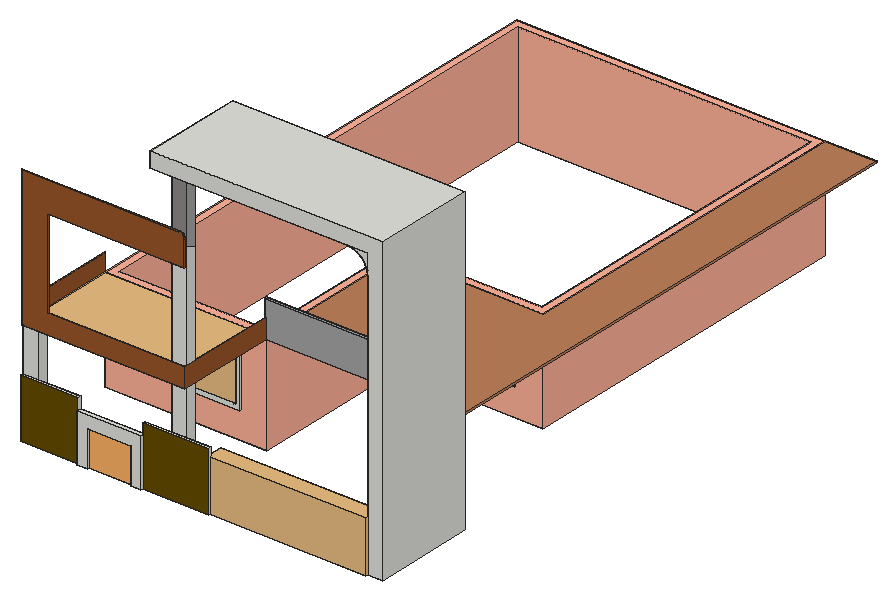
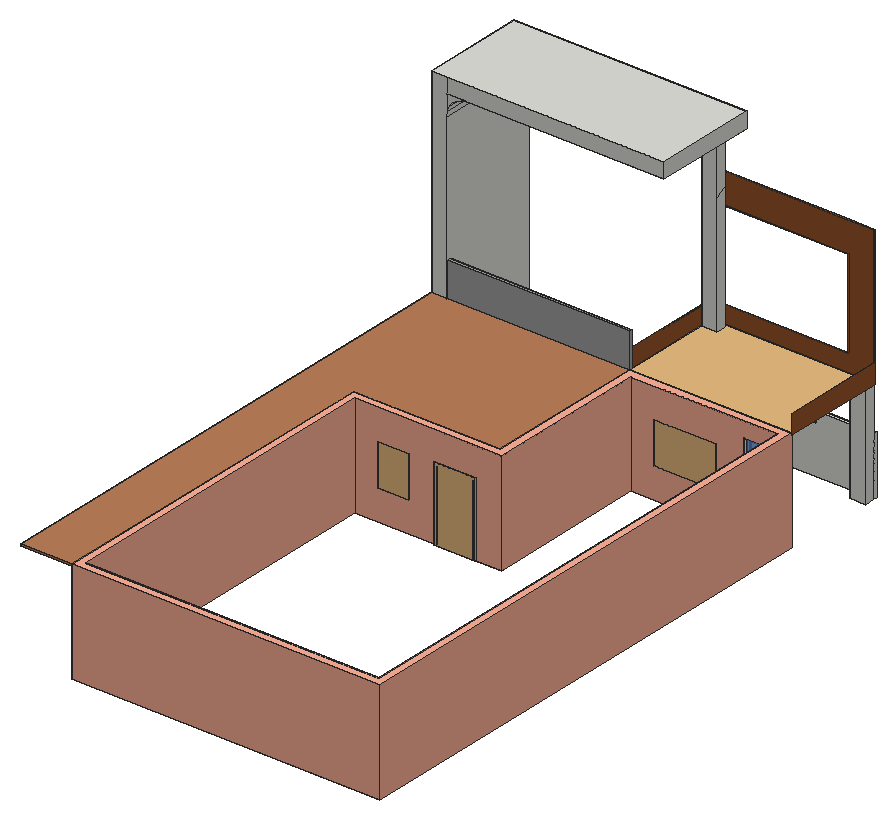
# SketchUp Ruby script. Lengths in inches.
U = 1.inch
M = Sketchup.active_model
def pt(a) = Geom::Point3d.new(a.map { |v| v * U })
def face(e, loops, mat)
  f = e.add_face(loops[0].map { |a| pt(a) })
  loops[1..].each { |l| e.add_face(l.map { |a| pt(a) }).erase! }
  f.material = f.back_material = mat if mat
  f
end
# faces: each face lists its corners as indices into pts; further lists are holes
def faces(e, pts, list, mat = nil) = list.each { |f| face(e, (f[0].is_a?(Array) ? f : [f]).map { |l| l.map { |i| pts[i] } }, mat) }
# xy, xz, yz: faces in a plane at the given z, y or x. An outline is a flat list of corners, or four numbers for a rectangle; further outlines are holes
def ring(l) = l.size == 4 ? [[l[0], l[1]], [l[2], l[1]], [l[2], l[3]], [l[0], l[3]]] : l.each_slice(2).to_a
def flat(e, list, mat, &to3) = list.each { |f| face(e, (f[0].is_a?(Array) ? f : [f]).map { |l| ring(l).map { |u, v| to3.(u, v) } }, mat) }
def xy(e, z, list, mat = nil) = flat(e, list, mat) { |x, y| [x, y, z] }
def xz(e, y, list, mat = nil) = flat(e, list, mat) { |x, z| [x, y, z] }
def yz(e, x, list, mat = nil) = flat(e, list, mat) { |y, z| [x, y, z] }
def lines(e, pts, list) = list.each { |a, b| e.add_line(pt(pts[a]), pt(pts[b])) }
# prism: a flat outline (further loops are holes) pulled along v
def prism(e, loops, v, mat = nil)
  f = face(e, loops, mat); d = Geom::Vector3d.new(v.map { |x| x * U })
  f.pushpull(f.normal.samedirection?(d) ? d.length : -d.length)
end
def box(e, o, s, mat = nil) = prism(e, [[o, [o[0] + s[0], o[1], o[2]], [o[0] + s[0], o[1] + s[1], o[2]], [o[0], o[1] + s[1], o[2]]]], [0, 0, s[2]], mat)
def at(x, y, z, deg = 0) = Geom::Transformation.translation(pt([x, y, z])) * Geom::Transformation.rotation(ORIGIN, Z_AXIS, deg.degrees)
def axes(o, x, y, z) = Geom::Transformation.new([*x, 0, *y, 0, *z, 0, *pt(o).to_a, 1])
def part(name) = M.definitions.add(name)
# library, detail: a bought-in or finely detailed component or shape, given as its bounding box
def library(name, o, s) = part(name).tap { |d| box(d.entities, o, s) }
def detail(e, o, s) = box(e.add_group.entities, o, s)
def put(e, d, t, mat = nil) = e.add_instance(d, t).tap { |i| i.material = mat if mat }
def group(e, t, mat = nil) = e.add_group.tap { |g| g.transformation = t; g.material = mat if mat }.entities
root = M.entities
M.materials.add("[Color B02]").color = [255, 178, 153]
M.materials.add("[Color B08]").color = [102, 25, 0]
M.materials.add("[Color C03]").color = [255, 178, 101]
M.materials.add("[Color D02]").color = [255, 229, 153]
M.materials.add("[Color D08]").color = [102, 76, 0]
M.materials.add("[Metal Silver]").color = [234, 233, 238]
M.materials.add("[Stone Marble]").color = [143, 138, 136]
M.materials.add("[Stone Vein Gray]").color = [166, 165, 165]
M.materials.add("[Translucent Glass Blue]").color = [100, 149, 237]
M.materials["[Translucent Glass Blue]"].alpha = 0.5
M.materials.add("[Wood Cherry Original]").color = [152, 86, 42]
M.materials.add("[Wood Veneer 02]").color = [190, 128, 91]
c1 = library("Main Gate",[0,-1.74,0],[119.75,5.32,60.06])
c2 = library("Group\#3",[0,0,0],[47.51,11.03,86.76])
c3 = part("Difference\#2")
xy(c3.entities,0,[[0,0,0,600,360,600,360,189,255,189,255,198,351,198,351,591,9,591,9,9,180,9,180,198,213,198,213,189,189,189,189,0]])
xy(c3.entities,36,[[81,0,153,9],[288,189,324,198]])
xy(c3.entities,78,[[24,0,48,9]])
xy(c3.entities,84,[[81,0,153,9],[213,189,255,198],[288,189,324,198]])
xy(c3.entities,102,[[24,0,48,9]])
xy(c3.entities,120,[[[0,0,189,0,189,189,360,189,360,600,0,600],[9,9,9,591,351,591,351,198,180,198,180,9]]])
xz(c3.entities,0,[[[0,0,189,120],[81,36,153,84],[24,78,48,102]]])
xz(c3.entities,9,[[[9,0,180,120],[81,36,153,84],[24,78,48,102]]])
xz(c3.entities,189,[[[189,0,213,0,213,84,255,84,255,0,360,0,360,120,189,120],[288,36,324,84]]])
xz(c3.entities,198,[[[180,0,180,120,351,120,351,0,255,0,255,84,213,84,213,0],[288,36,324,84]]])
xz(c3.entities,591,[[9,0,351,120]])
xz(c3.entities,600,[[0,0,360,120]])
yz(c3.entities,0,[[0,0,600,120]])
yz(c3.entities,9,[[9,0,591,120]])
yz(c3.entities,24,[[0,78,9,102]])
yz(c3.entities,48,[[0,78,9,102]])
yz(c3.entities,81,[[0,36,9,84]])
yz(c3.entities,153,[[0,36,9,84]])
yz(c3.entities,180,[[9,0,198,120]])
yz(c3.entities,189,[[0,0,189,120]])
yz(c3.entities,213,[[189,0,198,84]])
yz(c3.entities,255,[[189,0,198,84]])
yz(c3.entities,288,[[189,36,198,84]])
yz(c3.entities,324,[[189,36,198,84]])
yz(c3.entities,351,[[198,0,591,120]])
yz(c3.entities,360,[[189,0,600,120]])
c4 = part("Group\#9")
prism(c4.entities,[[[82.01,1,58.01],[82.01,1,0],[0,1,0],[0,1,58.01]],[[5.04,1,52.97],[5.04,1,5.04],[76.97,1,5.04],[76.97,1,52.97]]],[0,-1,0])
c5 = part("Group\#10")
prism(c5.entities,[[[42.49,0,54.49],[0,0,54.49],[0,0,0],[42.49,0,0]],[[3.28,0,51.21],[39.21,0,51.21],[39.21,0,3.28],[3.28,0,3.28]]],[0,1,0])
c6 = library("Group\#23",[0,0,0],[36,9.07,48])
c7 = library("Group\#22",[0,0,0],[72,9.07,48])
c8 = part("Group15\#2")
box(c8.entities,[1.02,2.16,1.02],[21.96,1.15,21.96])
c9 = part("Group\#7")
put(c9.entities,c8,at(0,0,0),"[Translucent Glass Blue]")
g1 = group(c9.entities,at(0,0,0),"[Metal Silver]")
xy(g1,0,[[0,0,24,9]])
xy(g1,0.83,[[0.83,4.61,23.17,8.93]])
xy(g1,1.02,[[1.02,2.16,22.98,3.3125]])
xy(g1,1.61,[[1.61,1.8,22.39,2.16]])
xy(g1,1.65,[[1.65,3.3125,22.35,3.46]])
xy(g1,22.35,[[1.65,3.3125,22.35,3.46]])
xy(g1,22.39,[[1.61,1.8,22.39,2.16]])
xy(g1,22.98,[[1.02,2.16,22.98,3.3125]])
xy(g1,23.17,[[0.83,4.61,23.17,8.93]])
xy(g1,24,[[0,0,24,9]])
xz(g1,0,[[[0,0,24,24],[0.39,0.39,23.61,23.61]]])
xz(g1,0.36,[[[0.59,0.59,23.41,23.41],[0.79,0.79,23.21,23.21]]])
xz(g1,1.8,[[[0.83,0.83,23.17,23.17],[1.61,1.61,22.39,22.39]]])
xz(g1,2.16,[[[1.02,1.02,22.98,22.98],[1.61,1.61,22.39,22.39]]])
xz(g1,3.3125,[[[1.02,1.02,22.98,22.98],[1.65,1.65,22.35,22.35]]])
xz(g1,4.61,[[[0.83,0.83,23.17,23.17],[1.5,1.5,22.5,22.5]]])
xz(g1,9.07,[[[0.04,0.04,23.96,23.96],[0.75,0.75,23.25,23.25]]])
yz(g1,0,[[0,0,9,24]])
yz(g1,0.83,[[4.61,0.83,8.93,23.17]])
yz(g1,1.02,[[2.16,1.02,3.3125,22.98]])
yz(g1,1.61,[[1.8,1.61,2.16,22.39]])
yz(g1,1.65,[[3.3125,1.65,3.46,22.35]])
yz(g1,22.35,[[3.3125,1.65,3.46,22.35]])
yz(g1,22.39,[[1.8,1.61,2.16,22.39]])
yz(g1,22.98,[[2.16,1.02,3.3125,22.98]])
yz(g1,23.17,[[4.61,0.83,8.93,23.17]])
yz(g1,24,[[0,0,9,24]])
p = [[0,9,24],[0.04,9.07,23.96],[0.04,9.07,0.04],[0,9,0],[12,9.07,0.04],[23.96,9.07,0.04],
  [24,9,0],[12,9,0],[23.96,9.07,23.96],[24,9,24],[0.59,0.36,23.41],[0.39,0,23.61],
  [0.39,0,0.39],[0.59,0.36,0.59],[12,0,0.39],[23.61,0,0.39],[23.41,0.36,0.59],[12,0.36,0.59],
  [23.61,0,23.61],[23.41,0.36,23.41],[0.75,9.07,23.25],[0.83,8.93,23.17],[0.83,8.93,0.83],[0.75,9.07,0.75],
  [12,8.93,0.83],[23.17,8.93,0.83],[23.25,9.07,0.75],[12,9.07,0.75],[23.17,8.93,23.17],[23.25,9.07,23.25],
  [0.83,1.8,23.17],[0.79,0.36,23.21],[0.79,0.36,0.79],[0.83,1.8,0.83],[12,0.36,0.79],[23.21,0.36,0.79],
  [23.17,1.8,0.83],[12,1.8,0.83],[23.21,0.36,23.21],[23.17,1.8,23.17],[1.5,4.61,22.5],[1.65,3.46,22.35],
  [1.65,3.46,1.65],[1.5,4.61,1.5],[12,3.46,1.65],[22.35,3.46,1.65],[22.5,4.61,1.5],[12,4.61,1.5],
  [22.35,3.46,22.35],[22.5,4.61,22.5]]
faces(g1,p,[[0,1,2,3],[4,5,6,7,3,2],[6,5,8,9],[10,11,12,13],[14,15,16,17,13,12],[16,15,18,19],[20,21,22,23],[24,25,26,27,23,22],
  [26,25,28,29],[30,31,32,33],[34,35,36,37,33,32],[36,35,38,39],[40,41,42,43],[44,45,46,47,43,42],[46,45,48,49],[49,48,41,40],
  [39,38,31,30],[29,28,21,20],[19,18,11,10],[9,8,1,0]])
c10 = library("Group\#21",[0,0,0],[189,120,2])
g2 = group(root,at(403,6,-2.27))
xy(g2,0,[[0,0,18,120]])
xy(g2,336,[[-253.5,0,-24,120]])
xy(g2,354,[[-253.5,0,18,120]])
xz(g2,0,[[0,0,18,0,18,354,-253.5,354,-253.5,336,0,336],[0,312,0,336,-24,336,-17.79,335.18,-12,332.78,-7.03,328.97,-3.22,324,-0.82,318.21]])
xz(g2,120,[[0,0,18,354],[0,312,-0.82,318.21,-3.22,324,-7.03,328.97,-12,332.78,-17.79,335.18,-24,336,0,336],[-253.5,336,0,354]])
yz(g2,-253.5,[[0,336,120,354]])
yz(g2,0,[[0,0,120,312]])
yz(g2,18,[[0,0,120,354]])
p = [[0,120,312],[0,0,312],[-0.82,0,318.21],[-0.82,120,318.21],[-3.22,0,324],[-3.22,120,324],
  [-7.03,0,328.97],[-7.03,120,328.97],[-12,0,332.78],[-12,120,332.78],[-17.79,0,335.18],[-17.79,120,335.18],
  [-24,0,336],[-24,120,336]]
faces(g2,p,[[0,1,2,3],[3,2,4,5],[5,4,6,7],[7,6,8,9],[9,8,10,11],[11,10,12,13]])
put(root,c1,axes([217.65,16.93,-2.27],[1.54782,0,0],[0,-3.7464,0],[0,0,1]))
g3 = group(root,at(1,6,-2))
box(g3,[0,0,0],[18,12,120])
g4 = group(root,at(172,9,-2))
xy(g4,0,[[0,0,18,12]])
xy(g4,336,[[0,0,18,12]])
xz(g4,0,[[0,0,18,267.1]])
xz(g4,0,[[0,267.1,18,336]],"[Stone Marble]")
xz(g4,12,[[0,0,18,336]])
yz(g4,0,[[0,0,0,267.1,12,261.32,12,0],[12,261.32,0,267.1,0,336,12,336]])
yz(g4,18,[[0,0,12,0,12,261.32,0,267.1]])
yz(g4,18,[[12,261.32,12,336,0,336,0,267.1]],"[Stone Vein Gray]")
p = [[16.24,-3,280.24],[-0.91,-4,282]]
lines(g4,p,[[0,1]])
g5 = group(root,at(1,0,-2))
xy(g5,0,[[67.58,0,67.58,2,0,2,0,6,219.47,6,219.47,2,142.6,2,142.6,0,130.24,0,130.24,2,80.31,2,80.31,0]])
xy(g5,41.625,[[80.31,0,130.24,2]])
xy(g5,55.8,[[67.58,0,142.6,6]])
xy(g5,68.68,[[0,2,67.58,6],[142.6,2,219.47,6]])
xz(g5,0,[[67.58,0,80.31,0,80.31,41.625,130.24,41.625,130.24,0,142.6,0,142.6,55.8,67.58,55.8]])
xz(g5,2,[[80.31,0,130.24,41.625]],"[Color C03]")
xz(g5,2,[[0,0,67.58,68.68],[142.6,0,219.47,68.68]],"[Color D08]")
xz(g5,6,[[0,0,0,68.68,67.58,68.68,67.58,55.8,142.6,55.8,142.6,68.68,219.47,68.68,219.47,0]])
yz(g5,0,[[2,0,6,68.68]])
yz(g5,67.58,[[0,0,2,55.8],[2,55.8,6,68.68]])
yz(g5,80.31,[[0,0,2,41.625]])
yz(g5,130.24,[[0,0,2,41.625]])
yz(g5,142.6,[[0,0,2,55.8],[2,55.8,6,68.68]])
yz(g5,219.47,[[2,0,6,68.68]])
put(root,c2,at(211.24,313.82,0))
put(root,c3,at(1,126,0),"[Color B02]")
put(root,c4,at(77,124.93,31))
put(root,c5,at(285.76,313.93,32.76))
put(root,c6,at(325,324,35.96,180),"[Color B08]")
put(root,c7,at(154,135,36,180))
put(root,c9,at(49,135,78,180))
g6 = group(root,at(190,126,118),"[Wood Veneer 02]")
xy(g6,0,[[[0,0,0,189,171,189,171,600,231,600,231,0],[52.68,26.08,54.24,26.19,55.72,26.71,57.02,27.58,58.04,28.77,58.73,30.18,59.02,31.72,58.91,33.28,58.4,34.76,57.52,36.06,56.33,37.08,54.92,37.76,53.38,38.06,51.82,37.95,50.34,37.43,49.05,36.56,48.02,35.37,47.34,33.96,47.04,32.42,47.15,30.86,47.67,29.38,48.55,28.08,49.73,27.06,51.14,26.375],[52.68,86.08,54.24,86.19,55.72,86.71,57.02,87.58,58.04,88.77,58.73,90.18,59.02,91.72,58.91,93.28,58.4,94.76,57.52,96.06,56.33,97.08,54.92,97.76,53.38,98.06,51.82,97.95,50.34,97.43,49.05,96.56,48.02,95.37,47.34,93.96,47.04,92.42,47.15,90.86,47.67,89.38,48.55,88.08,49.73,87.06,51.14,86.375],[52.68,146.08,54.24,146.19,55.72,146.71,57.02,147.58,58.04,148.77,58.73,150.18,59.02,151.72,58.91,153.28,58.4,154.76,57.52,156.06,56.33,157.08,54.92,157.76,53.38,158.06,51.82,157.95,50.34,157.43,49.05,156.56,48.02,155.37,47.34,153.96,47.04,152.42,47.15,150.86,47.67,149.38,48.55,148.08,49.73,147.06,51.14,146.375],[135.55,26.08,137.12,26.19,138.6,26.71,139.89,27.58,140.92,28.77,141.6,30.18,141.9,31.72,141.78,33.28,141.27,34.76,140.39,36.06,139.21,37.08,137.8,37.76,136.26,38.06,134.7,37.95,133.22,37.43,131.92,36.56,130.9,35.37,130.21,33.96,129.92,32.42,130.03,30.86,130.54,29.38,131.42,28.08,132.61,27.06,134.01,26.375],[135.55,86.08,137.12,86.19,138.6,86.71,139.89,87.58,140.92,88.77,141.6,90.18,141.9,91.72,141.78,93.28,141.27,94.76,140.39,96.06,139.21,97.08,137.8,97.76,136.26,98.06,134.7,97.95,133.22,97.43,131.92,96.56,130.9,95.37,130.21,93.96,129.92,92.42,130.03,90.86,130.54,89.38,131.42,88.08,132.61,87.06,134.01,86.375],[135.55,146.08,137.12,146.19,138.6,146.71,139.89,147.58,140.92,148.77,141.6,150.18,141.9,151.72,141.78,153.28,141.27,154.76,140.39,156.06,139.21,157.08,137.8,157.76,136.26,158.06,134.7,157.95,133.22,157.43,131.92,156.56,130.9,155.37,130.21,153.96,129.92,152.42,130.03,150.86,130.54,149.38,131.42,148.08,132.61,147.06,134.01,146.375]]])
xy(g6,0.5,[[52.68,26.08,51.14,26.375,49.73,27.06,48.55,28.08,47.67,29.38,47.15,30.86,47.04,32.42,47.34,33.96,48.02,35.37,49.05,36.56,50.34,37.43,51.82,37.95,53.38,38.06,54.92,37.76,56.33,37.08,57.52,36.06,58.4,34.76,58.91,33.28,59.02,31.72,58.73,30.18,58.04,28.77,57.02,27.58,55.72,26.71,54.24,26.19],[135.55,26.08,134.01,26.375,132.61,27.06,131.42,28.08,130.54,29.38,130.03,30.86,129.92,32.42,130.21,33.96,130.9,35.37,131.92,36.56,133.22,37.43,134.7,37.95,136.26,38.06,137.8,37.76,139.21,37.08,140.39,36.06,141.27,34.76,141.78,33.28,141.9,31.72,141.6,30.18,140.92,28.77,139.89,27.58,138.6,26.71,137.12,26.19],[52.68,86.08,51.14,86.375,49.73,87.06,48.55,88.08,47.67,89.38,47.15,90.86,47.04,92.42,47.34,93.96,48.02,95.37,49.05,96.56,50.34,97.43,51.82,97.95,53.38,98.06,54.92,97.76,56.33,97.08,57.52,96.06,58.4,94.76,58.91,93.28,59.02,91.72,58.73,90.18,58.04,88.77,57.02,87.58,55.72,86.71,54.24,86.19],[135.55,86.08,134.01,86.375,132.61,87.06,131.42,88.08,130.54,89.38,130.03,90.86,129.92,92.42,130.21,93.96,130.9,95.37,131.92,96.56,133.22,97.43,134.7,97.95,136.26,98.06,137.8,97.76,139.21,97.08,140.39,96.06,141.27,94.76,141.78,93.28,141.9,91.72,141.6,90.18,140.92,88.77,139.89,87.58,138.6,86.71,137.12,86.19],[52.68,146.08,51.14,146.375,49.73,147.06,48.55,148.08,47.67,149.38,47.15,150.86,47.04,152.42,47.34,153.96,48.02,155.37,49.05,156.56,50.34,157.43,51.82,157.95,53.38,158.06,54.92,157.76,56.33,157.08,57.52,156.06,58.4,154.76,58.91,153.28,59.02,151.72,58.73,150.18,58.04,148.77,57.02,147.58,55.72,146.71,54.24,146.19],
  [135.55,146.08,134.01,146.375,132.61,147.06,131.42,148.08,130.54,149.38,130.03,150.86,129.92,152.42,130.21,153.96,130.9,155.37,131.92,156.56,133.22,157.43,134.7,157.95,136.26,158.06,137.8,157.76,139.21,157.08,140.39,156.06,141.27,154.76,141.78,153.28,141.9,151.72,141.6,150.18,140.92,148.77,139.89,147.58,138.6,146.71,137.12,146.19]],"[Color D02]")
xy(g6,2,[[0,0,231,0,231,600,171,600,171,189,0,189]])
xz(g6,0,[[0,0,231,2]])
xz(g6,189,[[0,0,171,2]])
xz(g6,600,[[171,0,231,2]])
yz(g6,0,[[0,0,189,2]])
yz(g6,171,[[189,0,600,2]])
yz(g6,231,[[0,0,600,2]])
p = [[52.68,26.08,0],[51.14,26.375,0],[51.14,26.375,0.5],[52.68,26.08,0.5],[54.24,26.19,0],[54.24,26.19,0.5],
  [135.55,26.08,0],[134.01,26.375,0],[134.01,26.375,0.5],[135.55,26.08,0.5],[137.12,26.19,0],[137.12,26.19,0.5],
  [55.72,26.71,0],[55.72,26.71,0.5],[138.6,26.71,0],[138.6,26.71,0.5],[49.73,27.06,0],[49.73,27.06,0.5],
  [132.61,27.06,0],[132.61,27.06,0.5],[57.02,27.58,0],[57.02,27.58,0.5],[139.89,27.58,0],[139.89,27.58,0.5],
  [48.55,28.08,0],[48.55,28.08,0.5],[131.42,28.08,0],[131.42,28.08,0.5],[58.04,28.77,0],[58.04,28.77,0.5],
  [140.92,28.77,0],[140.92,28.77,0.5],[47.67,29.38,0],[47.67,29.38,0.5],[130.54,29.38,0],[130.54,29.38,0.5],
  [58.73,30.18,0],[58.73,30.18,0.5],[141.6,30.18,0],[141.6,30.18,0.5],[47.15,30.86,0],[47.15,30.86,0.5],
  [130.03,30.86,0],[130.03,30.86,0.5],[59.02,31.72,0],[59.02,31.72,0.5],[141.9,31.72,0],[141.9,31.72,0.5],
  [47.04,32.42,0],[47.04,32.42,0.5],[129.92,32.42,0],[129.92,32.42,0.5],[58.91,33.28,0],[58.91,33.28,0.5],
  [141.78,33.28,0],[141.78,33.28,0.5],[47.34,33.96,0],[47.34,33.96,0.5],[130.21,33.96,0],[130.21,33.96,0.5],
  [58.4,34.76,0],[58.4,34.76,0.5],[141.27,34.76,0],[141.27,34.76,0.5],[48.02,35.37,0],[48.02,35.37,0.5],
  [130.9,35.37,0],[130.9,35.37,0.5],[57.52,36.06,0],[57.52,36.06,0.5],[140.39,36.06,0],[140.39,36.06,0.5],
  [49.05,36.56,0],[49.05,36.56,0.5],[131.92,36.56,0],[131.92,36.56,0.5],[56.33,37.08,0],[56.33,37.08,0.5],
  [139.21,37.08,0],[139.21,37.08,0.5],[50.34,37.43,0],[50.34,37.43,0.5],[133.22,37.43,0],[133.22,37.43,0.5],
  [54.92,37.76,0],[54.92,37.76,0.5],[137.8,37.76,0],[137.8,37.76,0.5],[51.82,37.95,0],[51.82,37.95,0.5],
  [134.7,37.95,0],[134.7,37.95,0.5],[53.38,38.06,0],[53.38,38.06,0.5],[136.26,38.06,0],[136.26,38.06,0.5],
  [52.68,86.08,0],[51.14,86.375,0],[51.14,86.375,0.5],[52.68,86.08,0.5],[54.24,86.19,0],[54.24,86.19,0.5],
  [135.55,86.08,0],[134.01,86.375,0],[134.01,86.375,0.5],[135.55,86.08,0.5],[137.12,86.19,0],[137.12,86.19,0.5],
  [55.72,86.71,0],[55.72,86.71,0.5],[138.6,86.71,0],[138.6,86.71,0.5],[49.73,87.06,0],[49.73,87.06,0.5],
  [132.61,87.06,0],[132.61,87.06,0.5],[57.02,87.58,0],[57.02,87.58,0.5],[139.89,87.58,0],[139.89,87.58,0.5],
  [48.55,88.08,0],[48.55,88.08,0.5],[131.42,88.08,0],[131.42,88.08,0.5],[58.04,88.77,0],[58.04,88.77,0.5],
  [140.92,88.77,0],[140.92,88.77,0.5],[47.67,89.38,0],[47.67,89.38,0.5],[130.54,89.38,0],[130.54,89.38,0.5],
  [58.73,90.18,0],[58.73,90.18,0.5],[141.6,90.18,0],[141.6,90.18,0.5],[47.15,90.86,0],[47.15,90.86,0.5],
  [130.03,90.86,0],[130.03,90.86,0.5],[59.02,91.72,0],[59.02,91.72,0.5],[141.9,91.72,0],[141.9,91.72,0.5],
  [47.04,92.42,0],[47.04,92.42,0.5],[129.92,92.42,0],[129.92,92.42,0.5],[58.91,93.28,0],[58.91,93.28,0.5],
  [141.78,93.28,0],[141.78,93.28,0.5],[47.34,93.96,0],[47.34,93.96,0.5],[130.21,93.96,0],[130.21,93.96,0.5],
  [58.4,94.76,0],[58.4,94.76,0.5],[141.27,94.76,0],[141.27,94.76,0.5],[48.02,95.37,0],[48.02,95.37,0.5],
  [130.9,95.37,0],[130.9,95.37,0.5],[57.52,96.06,0],[57.52,96.06,0.5],[140.39,96.06,0],[140.39,96.06,0.5],
  [49.05,96.56,0],[49.05,96.56,0.5],[131.92,96.56,0],[131.92,96.56,0.5],[56.33,97.08,0],[56.33,97.08,0.5],
  [139.21,97.08,0],[139.21,97.08,0.5],[50.34,97.43,0],[50.34,97.43,0.5],[133.22,97.43,0],[133.22,97.43,0.5],
  [54.92,97.76,0],[54.92,97.76,0.5],[137.8,97.76,0],[137.8,97.76,0.5],[51.82,97.95,0],[51.82,97.95,0.5],
  [134.7,97.95,0],[134.7,97.95,0.5],[53.38,98.06,0],[53.38,98.06,0.5],[136.26,98.06,0],[136.26,98.06,0.5],
  [52.68,146.08,0],[51.14,146.375,0],[51.14,146.375,0.5],[52.68,146.08,0.5],[54.24,146.19,0],[54.24,146.19,0.5],
  [135.55,146.08,0],[134.01,146.375,0],[134.01,146.375,0.5],[135.55,146.08,0.5],[137.12,146.19,0],[137.12,146.19,0.5],
  [55.72,146.71,0],[55.72,146.71,0.5],[138.6,146.71,0],[138.6,146.71,0.5],[49.73,147.06,0],[49.73,147.06,0.5],
  [132.61,147.06,0],[132.61,147.06,0.5],[57.02,147.58,0],[57.02,147.58,0.5],[139.89,147.58,0],[139.89,147.58,0.5],
  [48.55,148.08,0],[48.55,148.08,0.5],[131.42,148.08,0],[131.42,148.08,0.5],[58.04,148.77,0],[58.04,148.77,0.5],
  [140.92,148.77,0],[140.92,148.77,0.5],[47.67,149.38,0],[47.67,149.38,0.5],[130.54,149.38,0],[130.54,149.38,0.5],
  [58.73,150.18,0],[58.73,150.18,0.5],[141.6,150.18,0],[141.6,150.18,0.5],[47.15,150.86,0],[47.15,150.86,0.5],
  [130.03,150.86,0],[130.03,150.86,0.5],[59.02,151.72,0],[59.02,151.72,0.5],[141.9,151.72,0],[141.9,151.72,0.5],
  [47.04,152.42,0],[47.04,152.42,0.5],[129.92,152.42,0],[129.92,152.42,0.5],[58.91,153.28,0],[58.91,153.28,0.5],
  [141.78,153.28,0],[141.78,153.28,0.5],[47.34,153.96,0],[47.34,153.96,0.5],[130.21,153.96,0],[130.21,153.96,0.5],
  [58.4,154.76,0],[58.4,154.76,0.5],[141.27,154.76,0],[141.27,154.76,0.5],[48.02,155.37,0],[48.02,155.37,0.5],
  [130.9,155.37,0],[130.9,155.37,0.5],[57.52,156.06,0],[57.52,156.06,0.5],[140.39,156.06,0],[140.39,156.06,0.5],
  [49.05,156.56,0],[49.05,156.56,0.5],[131.92,156.56,0],[131.92,156.56,0.5],[56.33,157.08,0],[56.33,157.08,0.5],
  [139.21,157.08,0],[139.21,157.08,0.5],[50.34,157.43,0],[50.34,157.43,0.5],[133.22,157.43,0],[133.22,157.43,0.5],
  [54.92,157.76,0],[54.92,157.76,0.5],[137.8,157.76,0],[137.8,157.76,0.5],[51.82,157.95,0],[51.82,157.95,0.5],
  [134.7,157.95,0],[134.7,157.95,0.5],[53.38,158.06,0],[53.38,158.06,0.5],[136.26,158.06,0],[136.26,158.06,0.5]]
faces(g6,p,[[0,1,2,3],[4,0,3,5],[6,7,8,9],[10,6,9,11],[12,4,5,13],[14,10,11,15],[1,16,17,2],[7,18,19,8],
  [20,12,13,21],[22,14,15,23],[16,24,25,17],[18,26,27,19],[28,20,21,29],[30,22,23,31],[24,32,33,25],[26,34,35,27],
  [36,28,29,37],[38,30,31,39],[32,40,41,33],[34,42,43,35],[44,36,37,45],[46,38,39,47],[40,48,49,41],[42,50,51,43],
  [52,44,45,53],[54,46,47,55],[48,56,57,49],[50,58,59,51],[60,52,53,61],[62,54,55,63],[56,64,65,57],[58,66,67,59],
  [68,60,61,69],[70,62,63,71],[64,72,73,65],[66,74,75,67],[76,68,69,77],[78,70,71,79],[72,80,81,73],[74,82,83,75],
  [84,76,77,85],[86,78,79,87],[80,88,89,81],[82,90,91,83],[92,84,85,93],[94,86,87,95],[88,92,93,89],[90,94,95,91],
  [96,97,98,99],[100,96,99,101],[102,103,104,105],[106,102,105,107],[108,100,101,109],[110,106,107,111],[97,112,113,98],[103,114,115,104],
  [116,108,109,117],[118,110,111,119],[112,120,121,113],[114,122,123,115],[124,116,117,125],[126,118,119,127],[120,128,129,121],[122,130,131,123],
  [132,124,125,133],[134,126,127,135],[128,136,137,129],[130,138,139,131],[140,132,133,141],[142,134,135,143],[136,144,145,137],[138,146,147,139],
  [148,140,141,149],[150,142,143,151],[144,152,153,145],[146,154,155,147],[156,148,149,157],[158,150,151,159],[152,160,161,153],[154,162,163,155],
  [164,156,157,165],[166,158,159,167],[160,168,169,161],[162,170,171,163],[172,164,165,173],[174,166,167,175],[168,176,177,169],[170,178,179,171],
  [180,172,173,181],[182,174,175,183],[176,184,185,177],[178,186,187,179],[188,180,181,189],[190,182,183,191],[184,188,189,185],[186,190,191,187],
  [192,193,194,195],[196,192,195,197],[198,199,200,201],[202,198,201,203],[204,196,197,205],[206,202,203,207],[193,208,209,194],[199,210,211,200],
  [212,204,205,213],[214,206,207,215],[208,216,217,209],[210,218,219,211],[220,212,213,221],[222,214,215,223],[216,224,225,217],[218,226,227,219],
  [228,220,221,229],[230,222,223,231],[224,232,233,225],[226,234,235,227],[236,228,229,237],[238,230,231,239],[232,240,241,233],[234,242,243,235],
  [244,236,237,245],[246,238,239,247],[240,248,249,241],[242,250,251,243],[252,244,245,253],[254,246,247,255],[248,256,257,249],[250,258,259,251],
  [260,252,253,261],[262,254,255,263],[256,264,265,257],[258,266,267,259],[268,260,261,269],[270,262,263,271],[264,272,273,265],[266,274,275,267],
  [276,268,269,277],[278,270,271,279],[272,280,281,273],[274,282,283,275],[284,276,277,285],[286,278,279,287],[280,284,285,281],[282,286,287,283]])
g7 = group(root,at(190,122,118),"[Stone Vein Gray]")
box(g7,[0,0,0],[213,4,42])
g8 = group(root,at(0,5,118),"[Wood Cherry Original]")
xy(g8,0,[[0,0,191,1],[0,1,1,121],[190,1,191,117]])
xy(g8,22.55,[[30.57,0,191,1],[0,1,1,121],[190,1,191,117]])
xy(g8,126,[[30.57,0,190,1]])
xy(g8,162,[[0,0,30.57,1],[30.57,0,184,1]])
xz(g8,0,[[0,0,191,0,191,22.55,30.57,22.55,30.57,126,190,126,190,156,189.8,157.55,189.2,159,188.24,160.24,187,161.2,185.55,161.8,184,162,0,162]])
xz(g8,1,[[0,22.55,1,126],[0,126,1,162]])
xz(g8,117,[[190,0,191,22.55]])
xz(g8,121,[[0,0,1,22.55]])
yz(g8,0,[[0,0,0,162,1,162,1,22.55,121,22.55,121,0]])
yz(g8,30.57,[[0,22.55,1,126]])
yz(g8,190,[[0,126,1,156]])
yz(g8,191,[[0,0,117,22.55]])
p = [[189.8,1,157.55],[189.8,0,157.55],[190,0,156],[190,1,156],[189.2,1,159],[189.2,0,159],
  [188.24,1,160.24],[188.24,0,160.24],[187,1,161.2],[187,0,161.2],[185.55,1,161.8],[185.55,0,161.8],
  [184,1,162],[184,0,162]]
faces(g8,p,[[0,1,2,3],[4,5,1,0],[6,7,5,4],[8,9,7,6],[10,11,9,8],[12,13,11,10]])
put(root,c10,at(1,6,118),"[Wood Veneer 02]")
